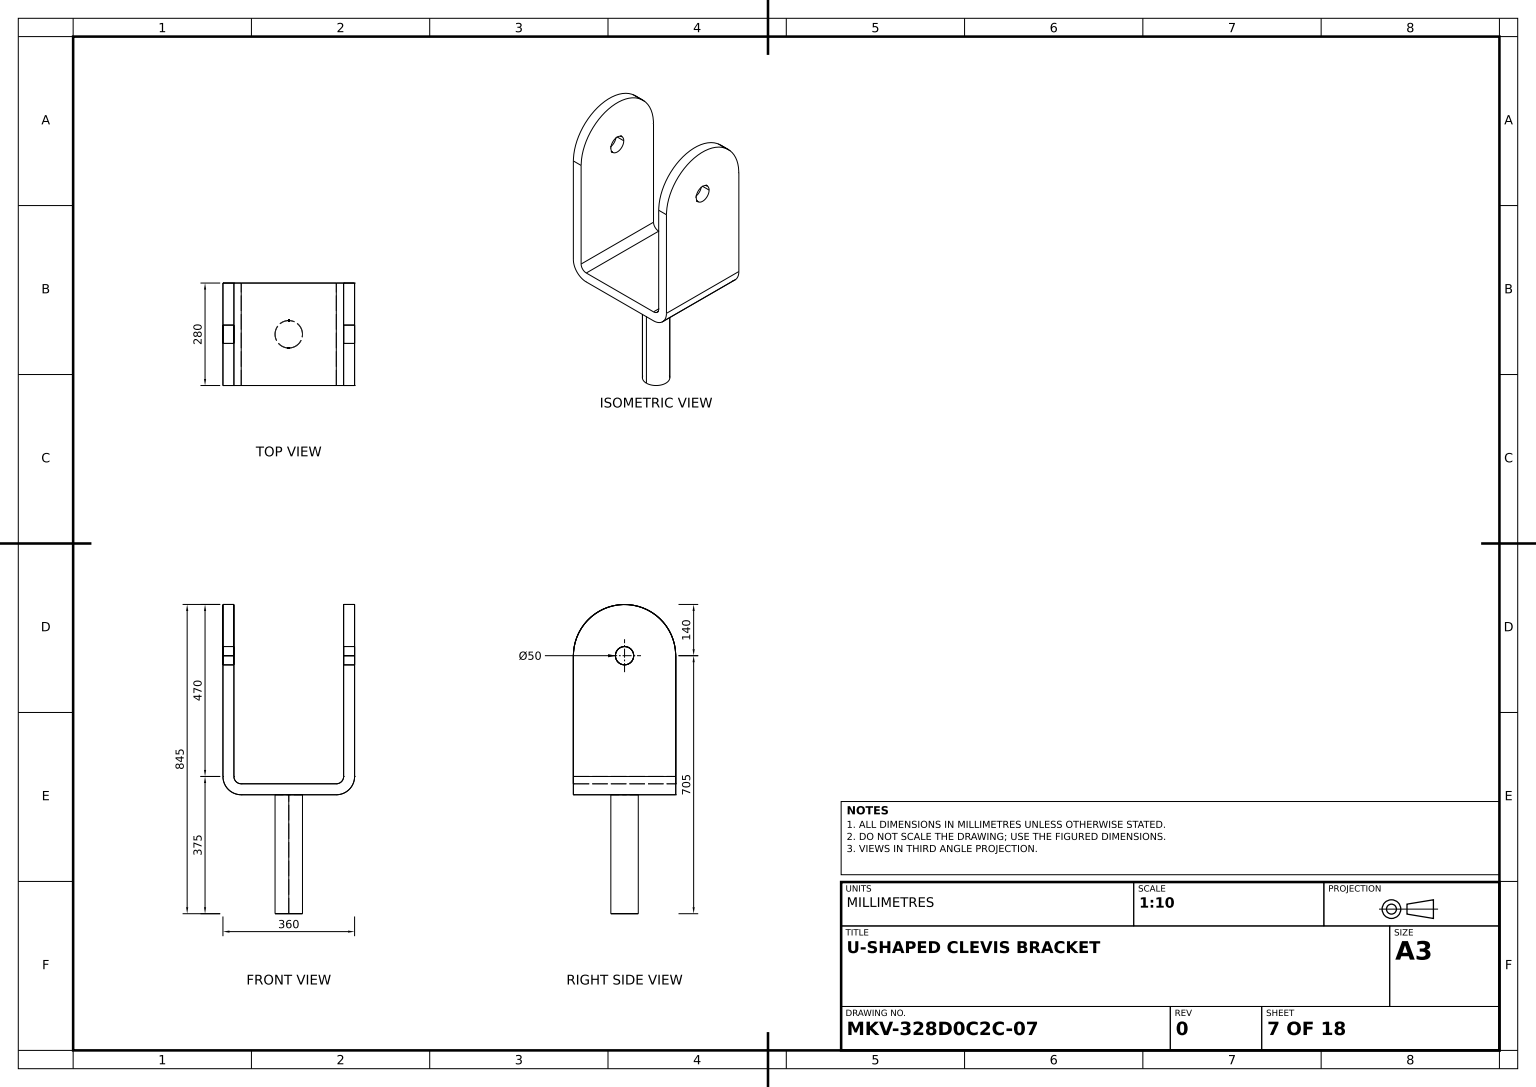
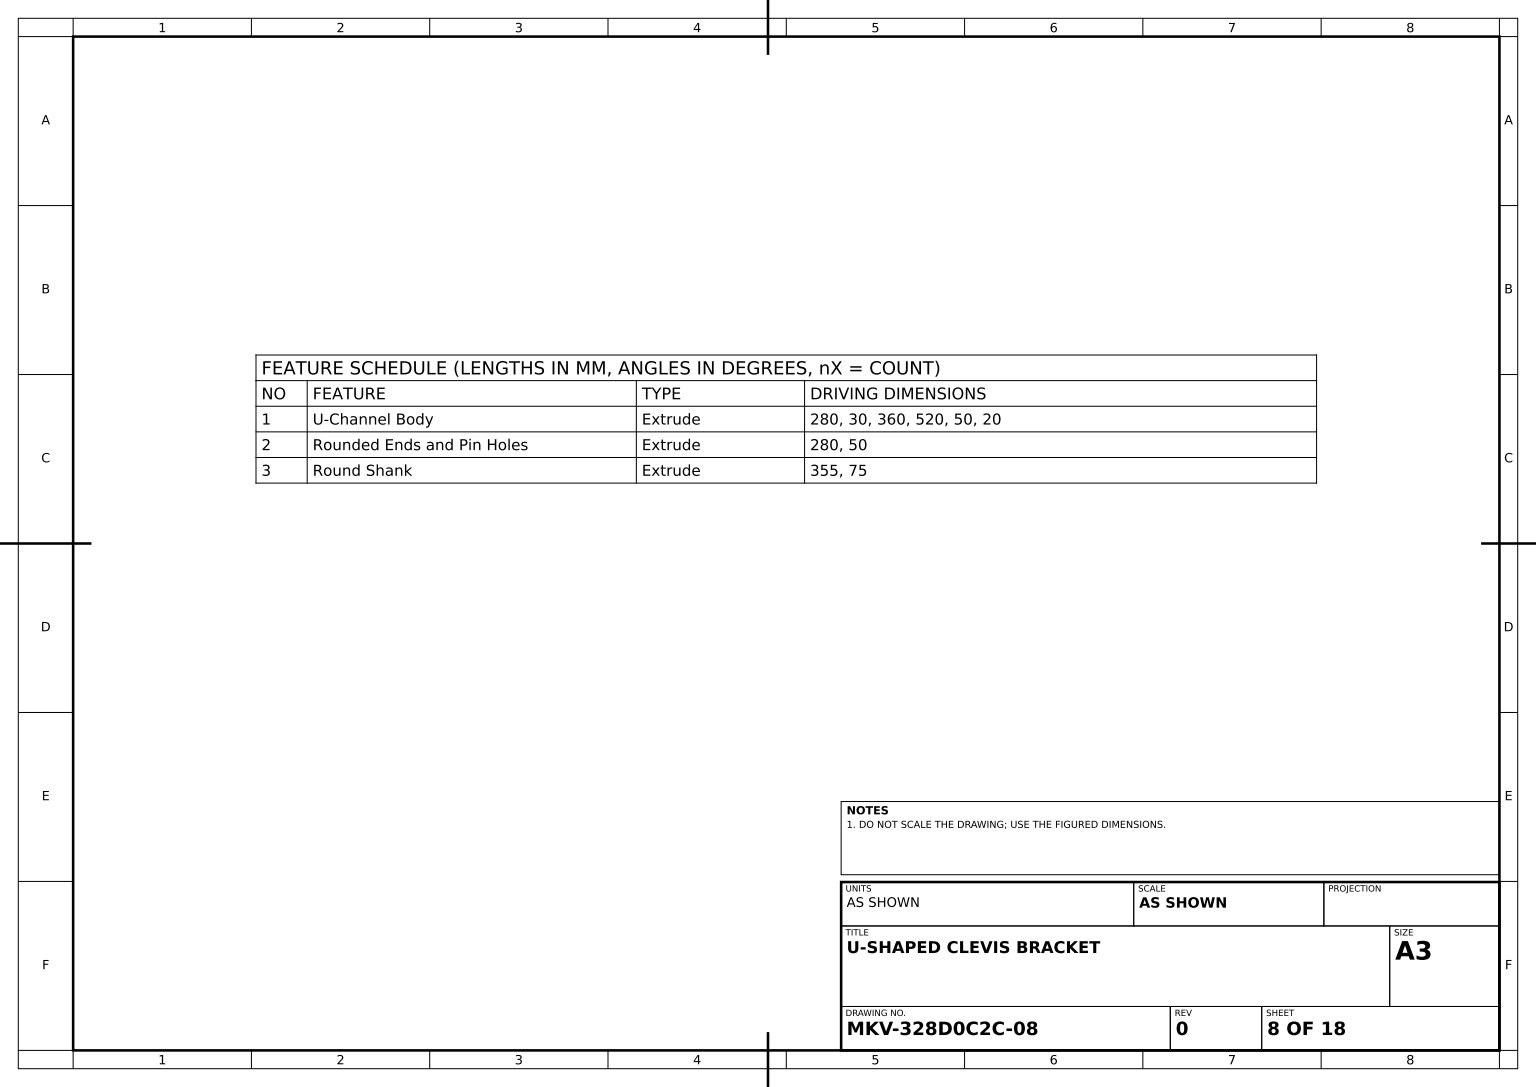
ISO-10303-21;
HEADER;
FILE_DESCRIPTION((''),'2;1');
FILE_NAME('','',(''),(''),'','','');
FILE_SCHEMA(('AUTOMOTIVE_DESIGN'));
ENDSEC;
DATA;
#1=APPLICATION_CONTEXT('');
#2=PRODUCT_CONTEXT('',#1,'mechanical');
#3=PRODUCT('','','',(#2));
#4=PRODUCT_DEFINITION_FORMATION('','',#3);
#5=PRODUCT_DEFINITION_CONTEXT('',#1,'design');
#6=PRODUCT_DEFINITION('','',#4,#5);
#7=PRODUCT_DEFINITION_SHAPE('','',#6);
#8=(LENGTH_UNIT()NAMED_UNIT(*)SI_UNIT(.MILLI.,.METRE.));
#9=(NAMED_UNIT(*)PLANE_ANGLE_UNIT()SI_UNIT($,.RADIAN.));
#10=(NAMED_UNIT(*)SI_UNIT($,.STERADIAN.)SOLID_ANGLE_UNIT());
#11=UNCERTAINTY_MEASURE_WITH_UNIT(LENGTH_MEASURE(1.E-05),#8,'distance_accuracy_value','');
#12=(GEOMETRIC_REPRESENTATION_CONTEXT(3)GLOBAL_UNCERTAINTY_ASSIGNED_CONTEXT((#11))GLOBAL_UNIT_ASSIGNED_CONTEXT((#8,#9,#10))REPRESENTATION_CONTEXT('',''));
#13=CARTESIAN_POINT('',(150.,50.,140.));
#14=VERTEX_POINT('',#13);
#15=CARTESIAN_POINT('',(130.,30.,140.));
#16=VERTEX_POINT('',#15);
#17=CARTESIAN_POINT('',(130.,50.,140.));
#18=DIRECTION('',(0.,0.,-1.));
#19=DIRECTION('',(-1.,0.,0.));
#20=AXIS2_PLACEMENT_3D('',#17,#18,#19);
#21=CIRCLE('',#20,20.);
#22=EDGE_CURVE('',#14,#16,#21,.T.);
#23=ORIENTED_EDGE('',*,*,#22,.F.);
#24=CARTESIAN_POINT('',(150.,50.,-140.));
#25=VERTEX_POINT('',#24);
#26=VECTOR('',#18,1000.);
#27=LINE('',#13,#26);
#28=EDGE_CURVE('',#14,#25,#27,.T.);
#29=ORIENTED_EDGE('',*,*,#28,.T.);
#30=CARTESIAN_POINT('',(130.,30.,-140.));
#31=VERTEX_POINT('',#30);
#32=CARTESIAN_POINT('',(130.,50.,-140.));
#33=AXIS2_PLACEMENT_3D('',#32,#18,#19);
#34=CIRCLE('',#33,20.);
#35=EDGE_CURVE('',#25,#31,#34,.T.);
#36=ORIENTED_EDGE('',*,*,#35,.T.);
#37=LINE('',#15,#26);
#38=EDGE_CURVE('',#16,#31,#37,.T.);
#39=ORIENTED_EDGE('',*,*,#38,.F.);
#40=EDGE_LOOP('',(#23,#29,#36,#39));
#41=FACE_OUTER_BOUND('',#40,.T.);
#42=CYLINDRICAL_SURFACE('',#20,20.);
#43=ADVANCED_FACE('',(#41),#42,.F.);
#44=CARTESIAN_POINT('',(-130.,0.,140.));
#45=VERTEX_POINT('',#44);
#46=CARTESIAN_POINT('',(-130.,0.,-140.));
#47=VERTEX_POINT('',#46);
#48=LINE('',#44,#26);
#49=EDGE_CURVE('',#45,#47,#48,.T.);
#50=ORIENTED_EDGE('',*,*,#49,.F.);
#51=CARTESIAN_POINT('',(-180.,50.,140.));
#52=VERTEX_POINT('',#51);
#53=CARTESIAN_POINT('',(-130.,50.,140.));
#54=DIRECTION('',(0.,0.,1.));
#55=DIRECTION('',(1.,0.,0.));
#56=AXIS2_PLACEMENT_3D('',#53,#54,#55);
#57=CIRCLE('',#56,50.);
#58=EDGE_CURVE('',#52,#45,#57,.T.);
#59=ORIENTED_EDGE('',*,*,#58,.F.);
#60=CARTESIAN_POINT('',(-180.,50.,-140.));
#61=VERTEX_POINT('',#60);
#62=LINE('',#51,#26);
#63=EDGE_CURVE('',#52,#61,#62,.T.);
#64=ORIENTED_EDGE('',*,*,#63,.T.);
#65=CARTESIAN_POINT('',(-130.,50.,-140.));
#66=AXIS2_PLACEMENT_3D('',#65,#54,#55);
#67=CIRCLE('',#66,50.);
#68=EDGE_CURVE('',#61,#47,#67,.T.);
#69=ORIENTED_EDGE('',*,*,#68,.T.);
#70=EDGE_LOOP('',(#50,#59,#64,#69));
#71=FACE_OUTER_BOUND('',#70,.T.);
#72=AXIS2_PLACEMENT_3D('',#53,#18,#19);
#73=CYLINDRICAL_SURFACE('',#72,50.);
#74=ADVANCED_FACE('',(#71),#73,.T.);
#75=CARTESIAN_POINT('',(-150.,380.,-25.));
#76=VERTEX_POINT('',#75);
#77=CARTESIAN_POINT('',(-150.,380.,25.));
#78=VERTEX_POINT('',#77);
#79=CARTESIAN_POINT('',(-150.,380.,0.));
#80=DIRECTION('',(0.,-1.,0.));
#81=AXIS2_PLACEMENT_3D('',#79,#19,#80);
#82=CIRCLE('',#81,25.);
#83=EDGE_CURVE('',#76,#78,#82,.T.);
#84=ORIENTED_EDGE('',*,*,#83,.F.);
#85=CARTESIAN_POINT('',(-180.,380.,-25.));
#86=VERTEX_POINT('',#85);
#87=VECTOR('',#55,1000.);
#88=LINE('',#85,#87);
#89=EDGE_CURVE('',#86,#76,#88,.T.);
#90=ORIENTED_EDGE('',*,*,#89,.F.);
#91=CARTESIAN_POINT('',(-180.,380.,25.));
#92=VERTEX_POINT('',#91);
#93=CARTESIAN_POINT('',(-180.,380.,0.));
#94=AXIS2_PLACEMENT_3D('',#93,#55,#18);
#95=CIRCLE('',#94,25.);
#96=EDGE_CURVE('',#92,#86,#95,.T.);
#97=ORIENTED_EDGE('',*,*,#96,.F.);
#98=LINE('',#91,#87);
#99=EDGE_CURVE('',#92,#78,#98,.T.);
#100=ORIENTED_EDGE('',*,*,#99,.T.);
#101=EDGE_LOOP('',(#84,#90,#97,#100));
#102=FACE_OUTER_BOUND('',#101,.T.);
#103=CYLINDRICAL_SURFACE('',#94,25.);
#104=ADVANCED_FACE('',(#102),#103,.F.);
#105=CARTESIAN_POINT('',(180.,380.,25.));
#106=VERTEX_POINT('',#105);
#107=CARTESIAN_POINT('',(180.,380.,-25.));
#108=VERTEX_POINT('',#107);
#109=CARTESIAN_POINT('',(180.,380.,0.));
#110=AXIS2_PLACEMENT_3D('',#109,#55,#18);
#111=CIRCLE('',#110,25.);
#112=EDGE_CURVE('',#106,#108,#111,.T.);
#113=ORIENTED_EDGE('',*,*,#112,.F.);
#114=EDGE_CURVE('',#108,#106,#111,.T.);
#115=ORIENTED_EDGE('',*,*,#114,.F.);
#116=EDGE_LOOP('',(#113,#115));
#117=FACE_BOUND('',#116,.T.);
#118=CARTESIAN_POINT('',(180.,380.,-140.));
#119=VERTEX_POINT('',#118);
#120=CARTESIAN_POINT('',(180.,380.,140.));
#121=VERTEX_POINT('',#120);
#122=CIRCLE('',#110,140.);
#123=EDGE_CURVE('',#119,#121,#122,.T.);
#124=ORIENTED_EDGE('',*,*,#123,.T.);
#125=CARTESIAN_POINT('',(180.,50.,140.));
#126=VERTEX_POINT('',#125);
#127=DIRECTION('',(0.,1.,0.));
#128=VECTOR('',#127,1000.);
#129=LINE('',#125,#128);
#130=EDGE_CURVE('',#126,#121,#129,.T.);
#131=ORIENTED_EDGE('',*,*,#130,.F.);
#132=CARTESIAN_POINT('',(180.,50.,-140.));
#133=VERTEX_POINT('',#132);
#134=LINE('',#125,#26);
#135=EDGE_CURVE('',#126,#133,#134,.T.);
#136=ORIENTED_EDGE('',*,*,#135,.T.);
#137=LINE('',#132,#128);
#138=EDGE_CURVE('',#133,#119,#137,.T.);
#139=ORIENTED_EDGE('',*,*,#138,.T.);
#140=EDGE_LOOP('',(#124,#131,#136,#139));
#141=FACE_OUTER_BOUND('',#140,.T.);
#142=AXIS2_PLACEMENT_3D('',#125,#19,#54);
#143=PLANE('',#142);
#144=ADVANCED_FACE('',(#117,#141),#143,.F.);
#145=CARTESIAN_POINT('',(130.,0.,140.));
#146=VERTEX_POINT('',#145);
#147=CARTESIAN_POINT('',(130.,0.,-140.));
#148=VERTEX_POINT('',#147);
#149=LINE('',#145,#26);
#150=EDGE_CURVE('',#146,#148,#149,.T.);
#151=ORIENTED_EDGE('',*,*,#150,.T.);
#152=AXIS2_PLACEMENT_3D('',#32,#54,#55);
#153=CIRCLE('',#152,50.);
#154=EDGE_CURVE('',#148,#133,#153,.T.);
#155=ORIENTED_EDGE('',*,*,#154,.T.);
#156=ORIENTED_EDGE('',*,*,#135,.F.);
#157=AXIS2_PLACEMENT_3D('',#17,#54,#55);
#158=CIRCLE('',#157,50.);
#159=EDGE_CURVE('',#146,#126,#158,.T.);
#160=ORIENTED_EDGE('',*,*,#159,.F.);
#161=EDGE_LOOP('',(#151,#155,#156,#160));
#162=FACE_OUTER_BOUND('',#161,.T.);
#163=CYLINDRICAL_SURFACE('',#20,50.);
#164=ADVANCED_FACE('',(#162),#163,.T.);
#165=CARTESIAN_POINT('',(150.,380.,-25.));
#166=VERTEX_POINT('',#165);
#167=CARTESIAN_POINT('',(150.,380.,25.));
#168=VERTEX_POINT('',#167);
#169=CARTESIAN_POINT('',(150.,380.,0.));
#170=AXIS2_PLACEMENT_3D('',#169,#55,#127);
#171=CIRCLE('',#170,25.);
#172=EDGE_CURVE('',#166,#168,#171,.T.);
#173=ORIENTED_EDGE('',*,*,#172,.T.);
#174=EDGE_CURVE('',#168,#166,#171,.T.);
#175=ORIENTED_EDGE('',*,*,#174,.T.);
#176=EDGE_LOOP('',(#173,#175));
#177=FACE_BOUND('',#176,.T.);
#178=CARTESIAN_POINT('',(150.,380.,-140.));
#179=VERTEX_POINT('',#178);
#180=CARTESIAN_POINT('',(150.,520.,-140.));
#181=VECTOR('',#80,1000.);
#182=LINE('',#180,#181);
#183=EDGE_CURVE('',#179,#25,#182,.T.);
#184=ORIENTED_EDGE('',*,*,#183,.T.);
#185=ORIENTED_EDGE('',*,*,#28,.F.);
#186=CARTESIAN_POINT('',(150.,380.,140.));
#187=VERTEX_POINT('',#186);
#188=CARTESIAN_POINT('',(150.,520.,140.));
#189=LINE('',#188,#181);
#190=EDGE_CURVE('',#187,#14,#189,.T.);
#191=ORIENTED_EDGE('',*,*,#190,.F.);
#192=CIRCLE('',#170,140.);
#193=EDGE_CURVE('',#179,#187,#192,.T.);
#194=ORIENTED_EDGE('',*,*,#193,.F.);
#195=EDGE_LOOP('',(#184,#185,#191,#194));
#196=FACE_OUTER_BOUND('',#195,.T.);
#197=AXIS2_PLACEMENT_3D('',#188,#55,#127);
#198=PLANE('',#197);
#199=ADVANCED_FACE('',(#177,#196),#198,.F.);
#200=ORIENTED_EDGE('',*,*,#172,.F.);
#201=EDGE_CURVE('',#166,#108,#88,.T.);
#202=ORIENTED_EDGE('',*,*,#201,.T.);
#203=ORIENTED_EDGE('',*,*,#114,.T.);
#204=EDGE_CURVE('',#168,#106,#98,.T.);
#205=ORIENTED_EDGE('',*,*,#204,.F.);
#206=EDGE_LOOP('',(#200,#202,#203,#205));
#207=FACE_OUTER_BOUND('',#206,.T.);
#208=ADVANCED_FACE('',(#207),#103,.F.);
#209=ORIENTED_EDGE('',*,*,#83,.T.);
#210=EDGE_CURVE('',#78,#76,#82,.T.);
#211=ORIENTED_EDGE('',*,*,#210,.T.);
#212=EDGE_LOOP('',(#209,#211));
#213=FACE_BOUND('',#212,.T.);
#214=CARTESIAN_POINT('',(-150.,50.,140.));
#215=VERTEX_POINT('',#214);
#216=CARTESIAN_POINT('',(-150.,50.,-140.));
#217=VERTEX_POINT('',#216);
#218=LINE('',#214,#26);
#219=EDGE_CURVE('',#215,#217,#218,.T.);
#220=ORIENTED_EDGE('',*,*,#219,.T.);
#221=CARTESIAN_POINT('',(-150.,380.,-140.));
#222=VERTEX_POINT('',#221);
#223=LINE('',#216,#128);
#224=EDGE_CURVE('',#217,#222,#223,.T.);
#225=ORIENTED_EDGE('',*,*,#224,.T.);
#226=CARTESIAN_POINT('',(-150.,380.,140.));
#227=VERTEX_POINT('',#226);
#228=CIRCLE('',#81,140.);
#229=EDGE_CURVE('',#227,#222,#228,.T.);
#230=ORIENTED_EDGE('',*,*,#229,.F.);
#231=LINE('',#214,#128);
#232=EDGE_CURVE('',#215,#227,#231,.T.);
#233=ORIENTED_EDGE('',*,*,#232,.F.);
#234=EDGE_LOOP('',(#220,#225,#230,#233));
#235=FACE_OUTER_BOUND('',#234,.T.);
#236=AXIS2_PLACEMENT_3D('',#214,#19,#80);
#237=PLANE('',#236);
#238=ADVANCED_FACE('',(#213,#235),#237,.F.);
#239=CARTESIAN_POINT('',(-180.,380.,-140.));
#240=LINE('',#239,#87);
#241=EDGE_CURVE('',#179,#119,#240,.T.);
#242=ORIENTED_EDGE('',*,*,#241,.F.);
#243=ORIENTED_EDGE('',*,*,#193,.T.);
#244=CARTESIAN_POINT('',(-180.,380.,140.));
#245=LINE('',#244,#87);
#246=EDGE_CURVE('',#187,#121,#245,.T.);
#247=ORIENTED_EDGE('',*,*,#246,.T.);
#248=ORIENTED_EDGE('',*,*,#123,.F.);
#249=EDGE_LOOP('',(#242,#243,#247,#248));
#250=FACE_OUTER_BOUND('',#249,.T.);
#251=CYLINDRICAL_SURFACE('',#94,140.);
#252=ADVANCED_FACE('',(#250),#251,.T.);
#253=CARTESIAN_POINT('',(-130.,30.,140.));
#254=VERTEX_POINT('',#253);
#255=CIRCLE('',#72,20.);
#256=EDGE_CURVE('',#254,#215,#255,.T.);
#257=ORIENTED_EDGE('',*,*,#256,.T.);
#258=ORIENTED_EDGE('',*,*,#232,.T.);
#259=VERTEX_POINT('',#244);
#260=EDGE_CURVE('',#259,#227,#245,.T.);
#261=ORIENTED_EDGE('',*,*,#260,.F.);
#262=CARTESIAN_POINT('',(-180.,520.,140.));
#263=LINE('',#262,#181);
#264=EDGE_CURVE('',#259,#52,#263,.T.);
#265=ORIENTED_EDGE('',*,*,#264,.T.);
#266=ORIENTED_EDGE('',*,*,#58,.T.);
#267=LINE('',#44,#87);
#268=EDGE_CURVE('',#45,#146,#267,.T.);
#269=ORIENTED_EDGE('',*,*,#268,.T.);
#270=ORIENTED_EDGE('',*,*,#159,.T.);
#271=ORIENTED_EDGE('',*,*,#130,.T.);
#272=ORIENTED_EDGE('',*,*,#246,.F.);
#273=ORIENTED_EDGE('',*,*,#190,.T.);
#274=ORIENTED_EDGE('',*,*,#22,.T.);
#275=VECTOR('',#19,1000.);
#276=LINE('',#15,#275);
#277=EDGE_CURVE('',#16,#254,#276,.T.);
#278=ORIENTED_EDGE('',*,*,#277,.T.);
#279=EDGE_LOOP('',(#257,#258,#261,#265,#266,#269,#270,#271,#272,#273,#274,#278));
#280=FACE_OUTER_BOUND('',#279,.T.);
#281=PLANE('',#56);
#282=ADVANCED_FACE('',(#280),#281,.T.);
#283=EDGE_CURVE('',#86,#92,#95,.T.);
#284=ORIENTED_EDGE('',*,*,#283,.T.);
#285=ORIENTED_EDGE('',*,*,#96,.T.);
#286=EDGE_LOOP('',(#284,#285));
#287=FACE_BOUND('',#286,.T.);
#288=ORIENTED_EDGE('',*,*,#63,.F.);
#289=ORIENTED_EDGE('',*,*,#264,.F.);
#290=VERTEX_POINT('',#239);
#291=CIRCLE('',#94,140.);
#292=EDGE_CURVE('',#290,#259,#291,.T.);
#293=ORIENTED_EDGE('',*,*,#292,.F.);
#294=CARTESIAN_POINT('',(-180.,520.,-140.));
#295=LINE('',#294,#181);
#296=EDGE_CURVE('',#290,#61,#295,.T.);
#297=ORIENTED_EDGE('',*,*,#296,.T.);
#298=EDGE_LOOP('',(#288,#289,#293,#297));
#299=FACE_OUTER_BOUND('',#298,.T.);
#300=AXIS2_PLACEMENT_3D('',#262,#55,#18);
#301=PLANE('',#300);
#302=ADVANCED_FACE('',(#287,#299),#301,.F.);
#303=ORIENTED_EDGE('',*,*,#174,.F.);
#304=ORIENTED_EDGE('',*,*,#204,.T.);
#305=ORIENTED_EDGE('',*,*,#112,.T.);
#306=ORIENTED_EDGE('',*,*,#201,.F.);
#307=EDGE_LOOP('',(#303,#304,#305,#306));
#308=FACE_OUTER_BOUND('',#307,.T.);
#309=ADVANCED_FACE('',(#308),#103,.F.);
#310=CARTESIAN_POINT('',(0.,-325.,37.5));
#311=VERTEX_POINT('',#310);
#312=CARTESIAN_POINT('',(0.,-325.,-37.5));
#313=VERTEX_POINT('',#312);
#314=CARTESIAN_POINT('',(0.,-325.,0.));
#315=AXIS2_PLACEMENT_3D('',#314,#127,#54);
#316=CIRCLE('',#315,37.5);
#317=EDGE_CURVE('',#311,#313,#316,.T.);
#318=ORIENTED_EDGE('',*,*,#317,.F.);
#319=EDGE_CURVE('',#313,#311,#316,.T.);
#320=ORIENTED_EDGE('',*,*,#319,.F.);
#321=EDGE_LOOP('',(#318,#320));
#322=FACE_OUTER_BOUND('',#321,.T.);
#323=PLANE('',#315);
#324=ADVANCED_FACE('',(#322),#323,.F.);
#325=ORIENTED_EDGE('',*,*,#319,.T.);
#326=CARTESIAN_POINT('',(0.,0.,37.5));
#327=VERTEX_POINT('',#326);
#328=LINE('',#310,#128);
#329=EDGE_CURVE('',#311,#327,#328,.T.);
#330=ORIENTED_EDGE('',*,*,#329,.T.);
#331=CARTESIAN_POINT('',(0.,0.,-37.5));
#332=VERTEX_POINT('',#331);
#333=CARTESIAN_POINT('',(0.,0.,0.));
#334=AXIS2_PLACEMENT_3D('',#333,#127,#54);
#335=CIRCLE('',#334,37.5);
#336=EDGE_CURVE('',#332,#327,#335,.T.);
#337=ORIENTED_EDGE('',*,*,#336,.F.);
#338=LINE('',#312,#128);
#339=EDGE_CURVE('',#313,#332,#338,.T.);
#340=ORIENTED_EDGE('',*,*,#339,.F.);
#341=EDGE_LOOP('',(#325,#330,#337,#340));
#342=FACE_OUTER_BOUND('',#341,.T.);
#343=CYLINDRICAL_SURFACE('',#315,37.5);
#344=ADVANCED_FACE('',(#342),#343,.T.);
#345=ORIENTED_EDGE('',*,*,#317,.T.);
#346=ORIENTED_EDGE('',*,*,#339,.T.);
#347=EDGE_CURVE('',#327,#332,#335,.T.);
#348=ORIENTED_EDGE('',*,*,#347,.F.);
#349=ORIENTED_EDGE('',*,*,#329,.F.);
#350=EDGE_LOOP('',(#345,#346,#348,#349));
#351=FACE_OUTER_BOUND('',#350,.T.);
#352=ADVANCED_FACE('',(#351),#343,.T.);
#353=ORIENTED_EDGE('',*,*,#38,.T.);
#354=CARTESIAN_POINT('',(-130.,30.,-140.));
#355=VERTEX_POINT('',#354);
#356=LINE('',#30,#275);
#357=EDGE_CURVE('',#31,#355,#356,.T.);
#358=ORIENTED_EDGE('',*,*,#357,.T.);
#359=LINE('',#253,#26);
#360=EDGE_CURVE('',#254,#355,#359,.T.);
#361=ORIENTED_EDGE('',*,*,#360,.F.);
#362=ORIENTED_EDGE('',*,*,#277,.F.);
#363=EDGE_LOOP('',(#353,#358,#361,#362));
#364=FACE_OUTER_BOUND('',#363,.T.);
#365=AXIS2_PLACEMENT_3D('',#15,#80,#18);
#366=PLANE('',#365);
#367=ADVANCED_FACE('',(#364),#366,.F.);
#368=AXIS2_PLACEMENT_3D('',#65,#18,#19);
#369=CIRCLE('',#368,20.);
#370=EDGE_CURVE('',#355,#217,#369,.T.);
#371=ORIENTED_EDGE('',*,*,#370,.T.);
#372=ORIENTED_EDGE('',*,*,#219,.F.);
#373=ORIENTED_EDGE('',*,*,#256,.F.);
#374=ORIENTED_EDGE('',*,*,#360,.T.);
#375=EDGE_LOOP('',(#371,#372,#373,#374));
#376=FACE_OUTER_BOUND('',#375,.T.);
#377=CYLINDRICAL_SURFACE('',#72,20.);
#378=ADVANCED_FACE('',(#376),#377,.F.);
#379=ORIENTED_EDGE('',*,*,#347,.T.);
#380=ORIENTED_EDGE('',*,*,#336,.T.);
#381=EDGE_LOOP('',(#379,#380));
#382=FACE_BOUND('',#381,.T.);
#383=ORIENTED_EDGE('',*,*,#49,.T.);
#384=LINE('',#46,#87);
#385=EDGE_CURVE('',#47,#148,#384,.T.);
#386=ORIENTED_EDGE('',*,*,#385,.T.);
#387=ORIENTED_EDGE('',*,*,#150,.F.);
#388=ORIENTED_EDGE('',*,*,#268,.F.);
#389=EDGE_LOOP('',(#383,#386,#387,#388));
#390=FACE_OUTER_BOUND('',#389,.T.);
#391=AXIS2_PLACEMENT_3D('',#44,#127,#54);
#392=PLANE('',#391);
#393=ADVANCED_FACE('',(#382,#390),#392,.F.);
#394=EDGE_CURVE('',#290,#222,#240,.T.);
#395=ORIENTED_EDGE('',*,*,#394,.T.);
#396=ORIENTED_EDGE('',*,*,#224,.F.);
#397=ORIENTED_EDGE('',*,*,#370,.F.);
#398=ORIENTED_EDGE('',*,*,#357,.F.);
#399=ORIENTED_EDGE('',*,*,#35,.F.);
#400=ORIENTED_EDGE('',*,*,#183,.F.);
#401=ORIENTED_EDGE('',*,*,#241,.T.);
#402=ORIENTED_EDGE('',*,*,#138,.F.);
#403=ORIENTED_EDGE('',*,*,#154,.F.);
#404=ORIENTED_EDGE('',*,*,#385,.F.);
#405=ORIENTED_EDGE('',*,*,#68,.F.);
#406=ORIENTED_EDGE('',*,*,#296,.F.);
#407=EDGE_LOOP('',(#395,#396,#397,#398,#399,#400,#401,#402,#403,#404,#405,#406));
#408=FACE_OUTER_BOUND('',#407,.T.);
#409=PLANE('',#66);
#410=ADVANCED_FACE('',(#408),#409,.F.);
#411=ORIENTED_EDGE('',*,*,#210,.F.);
#412=ORIENTED_EDGE('',*,*,#99,.F.);
#413=ORIENTED_EDGE('',*,*,#283,.F.);
#414=ORIENTED_EDGE('',*,*,#89,.T.);
#415=EDGE_LOOP('',(#411,#412,#413,#414));
#416=FACE_OUTER_BOUND('',#415,.T.);
#417=ADVANCED_FACE('',(#416),#103,.F.);
#418=ORIENTED_EDGE('',*,*,#229,.T.);
#419=ORIENTED_EDGE('',*,*,#394,.F.);
#420=ORIENTED_EDGE('',*,*,#292,.T.);
#421=ORIENTED_EDGE('',*,*,#260,.T.);
#422=EDGE_LOOP('',(#418,#419,#420,#421));
#423=FACE_OUTER_BOUND('',#422,.T.);
#424=ADVANCED_FACE('',(#423),#251,.T.);
#425=CLOSED_SHELL('',(#43,#74,#104,#144,#164,#199,#208,#238,#252,#282,#302,#309,#324,#344,#352,#367,#378,#393,#410,#417,#424));
#426=MANIFOLD_SOLID_BREP('',#425);
#427=ADVANCED_BREP_SHAPE_REPRESENTATION('',(#426),#12);
#428=SHAPE_DEFINITION_REPRESENTATION(#7,#427);
ENDSEC;
END-ISO-10303-21;
